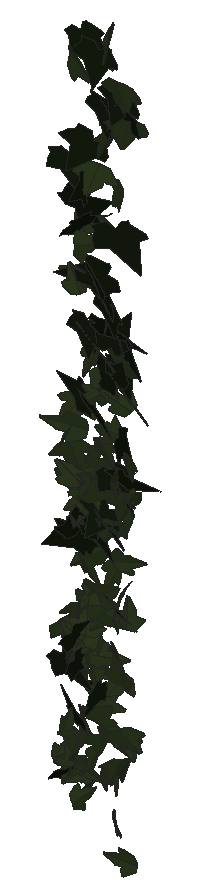
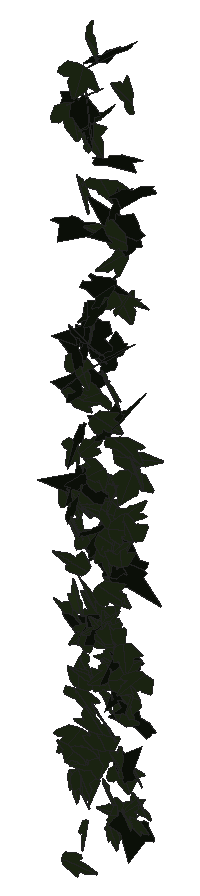
# SketchUp Ruby script. Lengths in inches.
U = 1.inch
M = Sketchup.active_model
def pt(a) = Geom::Point3d.new(a.map { |v| v * U })
def face(e, loops, mat)
  f = e.add_face(loops[0].map { |a| pt(a) })
  loops[1..].each { |l| e.add_face(l.map { |a| pt(a) }).erase! }
  f.material = f.back_material = mat if mat
  f
end
# faces: each face lists its corners as indices into pts; further lists are holes
def faces(e, pts, list, mat = nil) = list.each { |f| face(e, (f[0].is_a?(Array) ? f : [f]).map { |l| l.map { |i| pts[i] } }, mat) }
# xy, xz, yz: faces in a plane at the given z, y or x. An outline is a flat list of corners, or four numbers for a rectangle; further outlines are holes
def ring(l) = l.size == 4 ? [[l[0], l[1]], [l[2], l[1]], [l[2], l[3]], [l[0], l[3]]] : l.each_slice(2).to_a
def flat(e, list, mat, &to3) = list.each { |f| face(e, (f[0].is_a?(Array) ? f : [f]).map { |l| ring(l).map { |u, v| to3.(u, v) } }, mat) }
def xy(e, z, list, mat = nil) = flat(e, list, mat) { |x, y| [x, y, z] }
def xz(e, y, list, mat = nil) = flat(e, list, mat) { |x, z| [x, y, z] }
def yz(e, x, list, mat = nil) = flat(e, list, mat) { |y, z| [x, y, z] }
def lines(e, pts, list) = list.each { |a, b| e.add_line(pt(pts[a]), pt(pts[b])) }
# prism: a flat outline (further loops are holes) pulled along v
def prism(e, loops, v, mat = nil)
  f = face(e, loops, mat); d = Geom::Vector3d.new(v.map { |x| x * U })
  f.pushpull(f.normal.samedirection?(d) ? d.length : -d.length)
end
def box(e, o, s, mat = nil) = prism(e, [[o, [o[0] + s[0], o[1], o[2]], [o[0] + s[0], o[1] + s[1], o[2]], [o[0], o[1] + s[1], o[2]]]], [0, 0, s[2]], mat)
def at(x, y, z, deg = 0) = Geom::Transformation.translation(pt([x, y, z])) * Geom::Transformation.rotation(ORIGIN, Z_AXIS, deg.degrees)
def axes(o, x, y, z) = Geom::Transformation.new([*x, 0, *y, 0, *z, 0, *pt(o).to_a, 1])
def part(name) = M.definitions.add(name)
# library, detail: a bought-in or finely detailed component or shape, given as its bounding box
def library(name, o, s) = part(name).tap { |d| box(d.entities, o, s) }
def detail(e, o, s) = box(e.add_group.entities, o, s)
def put(e, d, t, mat = nil) = e.add_instance(d, t).tap { |i| i.material = mat if mat }
def group(e, t, mat = nil) = e.add_group.tap { |g| g.transformation = t; g.material = mat if mat }.entities
root = M.entities
M.materials.add("1026 AP 7946 SUNNY SIDE UP").color = [254, 231, 186]
M.materials.add("efeu1").color = [18, 25, 13]
M.materials.add("efeu2").color = [43, 57, 29]
c1 = part("ivyleaf_10")
p = [[0,0.5,-0.03],[-0.0625,2.02,-0.43],[-0.19,2.01,-0.46],[-0.54,1.05,-0.29],[-0.52,0.625,-0.18],[-0.83,0.76,-0.28],
  [-1.16,0.64,-0.33],[-1.15,0.33,-0.24],[-0.77,-0.39,0.02],[-0.3,-0.51,0.16],[0.04,-0.48,0.23],[-0.02,2.01,-0.4375],
  [-0.06,2.01,-0.43],[0.04,-0.49,0.23],[0.67,-0.49,0.14],[1.38,0.36,-0.2],[1.375,0.51,-0.24],[0.81,0.65,-0.19],
  [0.62,0.59,-0.15],[0.6,1.09,-0.28],[0.5,1.23,-0.31]]
faces(c1.entities,p,[[0,1,2,3,4,5,6,7,8,9,10],[11,12,0,13,14,15,16,17,18,19,20]],"efeu2")
c2 = part("ivyleaf_9")
p = [[1.54,2.16,1.25],[1.36,2.04,1.19],[-0.21,0.99,0.68],[-0.71,1.11,0.82],[-0.85,0.86,0.67],[-0.8,0.17,0.21],
  [-0.9,-0.01,0.1],[-0.67,-0.16,-0.02],[-0.08,-0.08,-0.05],[-0.03,-0.6,-0.4],[0.65,-0.88,-0.66],[0.83,-0.6,-0.49],
  [1.29,-0.42,-0.43],[1.8125,-0.07,-0.26],[1.21,0.44,0.15]]
faces(c2.entities,p,[[0,1,2,3,4,5,6,7,8,9,10,11,12,13,14]],"efeu1")
put(root,c1,axes([105.1,211.89,253.92],[0.25235,0.11815,0.14654],[-0.20286,-0.06215,0.20373],[0.20716,-0.20478,0.021]),"1026 AP 7946 SUNNY SIDE UP")
put(root,c2,axes([105.58,212.04,261.6],[0.04044,-0.21358,0.12299],[0.03918,-0.11835,-0.22211],[0.38367,0.0346,0.00972]),"1026 AP 7946 SUNNY SIDE UP")
put(root,c1,axes([105.06,211.72,250.5],[0.04226,0.045,-0.22259],[0.13994,0.19725,0.05482],[0.31799,-0.09279,0.00546]),"1026 AP 7946 SUNNY SIDE UP")
put(root,c2,axes([105.01,212.1,264.14],[0.00338,-0.11899,-0.23068],[0.24471,-0.17538,0.09682],[-0.31359,-0.13814,0.07306]),"1026 AP 7946 SUNNY SIDE UP")
put(root,c2,axes([105.33,212.05,267.23],[-0.1183,-0.24887,0.03019],[-0.00256,-0.03158,-0.26792],[0.39429,-0.07487,0.00732]),"1026 AP 7946 SUNNY SIDE UP")
put(root,c1,axes([104.97,211.93,251.83],[-0.2425,-0.13537,0.05546],[-0.04371,-0.05074,-0.21078],[0.22531,-0.15553,0.01879]),"1026 AP 7946 SUNNY SIDE UP")
put(root,c2,axes([105.14,212.04,259.25],[0.14991,-0.20524,0.14852],[0.09569,-0.13198,-0.23391],[0.38369,0.1131,0.00031]),"1026 AP 7946 SUNNY SIDE UP")
put(root,c2,axes([105.05,211.7,253.64],[0.00214,0.02141,-0.26801],[-0.22141,0.21927,0.01911],[0.34584,0.14024,0.01389]),"1026 AP 7946 SUNNY SIDE UP")
put(root,c2,axes([105.06,212.02,260.77],[0.20564,-0.18783,0.15192],[0.11526,-0.12971,-0.23623],[0.35845,0.14946,-0.01119]),"1026 AP 7946 SUNNY SIDE UP")
put(root,c2,axes([105.01,211.6875,263.38],[-0.03504,0.16493,-0.20943],[-0.03822,0.20278,0.17263],[0.41099,0.03292,-0.0018]),"1026 AP 7946 SUNNY SIDE UP")
put(root,c1,axes([104.89,211.97,258.68],[-0.0191,-0.02213,-0.2696],[-0.40694,-0.0428,0.01586],[-0.06906,0.25833,-0.0189]),"1026 AP 7946 SUNNY SIDE UP")
put(root,c1,axes([106,211.91,253.4],[-0.34779,0.05606,0.00791],[0.0193,0.0186,0.23418],[0.08678,0.22052,-0.02038]),"1026 AP 7946 SUNNY SIDE UP")
put(root,c1,axes([104.98,212,253.76],[0.20662,-0.06765,0.16385],[0.21278,-0.08479,-0.15246],[0.16995,0.1884,-0.00832]),"1026 AP 7946 SUNNY SIDE UP")
put(root,c1,axes([105.53,211.91,251.98],[-0.14705,-0.1867,-0.00857],[0.01832,0.00228,-0.21489],[0.29322,-0.09377,0.00913]),"1026 AP 7946 SUNNY SIDE UP")
put(root,c1,axes([105.96,211.76,257.87],[-0.04314,0.07268,0.21227],[-0.16295,0.17802,-0.07802],[-0.30176,-0.10653,0.01179]),"1026 AP 7946 SUNNY SIDE UP")
put(root,c1,axes([105.38,211.97,257.29],[-0.19438,-0.17108,-0.05241],[-0.06417,-0.03195,0.21678],[-0.27277,0.12943,-0.01365]),"1026 AP 7946 SUNNY SIDE UP")
put(root,c1,axes([104.66,211.9375,258.58],[0.12642,-0.22668,-0.02526],[-0.02371,0.01929,-0.24754],[0.35751,0.08143,-0.00749]),"1026 AP 7946 SUNNY SIDE UP")
put(root,c1,axes([106.25,211.89,249.42],[0.02755,-0.03254,-0.21439],[-0.31292,0.0653,-0.02742],[0.10763,0.19817,-0.02485]),"1026 AP 7946 SUNNY SIDE UP")
put(root,c2,axes([104.96,211.74,254.19],[-0.02593,0.01274,-0.26475],[-0.12622,0.24449,0.01922],[0.38452,0.08111,-0.01154]),"1026 AP 7946 SUNNY SIDE UP")
put(root,c2,axes([105.04,212.03,259.33],[0.03465,-0.26593,0.03037],[0.0179,0.032,0.27471],[-0.4206,-0.02054,0.01419]),"1026 AP 7946 SUNNY SIDE UP")
put(root,c1,axes([105.92,211.85,250.26],[-0.17709,0.1531,0.09478],[-0.10417,0.0641,-0.19491],[-0.26007,-0.12993,0.01353]),"1026 AP 7946 SUNNY SIDE UP")
put(root,c1,axes([105.19,212.1,254.97],[-0.0668,-0.06614,0.21725],[0.07074,-0.21321,-0.06069],[0.34082,0.03129,0.05518]),"1026 AP 7946 SUNNY SIDE UP")
put(root,c1,axes([105.68,211.81,251.22],[-0.05996,0.13436,0.16187],[-0.10001,0.14359,-0.14225],[-0.30835,-0.0727,0.01466]),"1026 AP 7946 SUNNY SIDE UP")
put(root,c1,axes([105.11,212,257.15],[0.24628,0.03322,-0.1483],[-0.21677,-0.04332,-0.16486],[-0.08432,0.2084,-0.00933]),"1026 AP 7946 SUNNY SIDE UP")
put(root,c2,axes([105.89,212.04,259.89],[0.23114,-0.19279,0.10579],[0.07883,-0.09205,-0.24984],[0.33513,0.15462,-0.0142]),"1026 AP 7946 SUNNY SIDE UP")
put(root,c1,axes([106.14,212.01,257.51],[-0.13584,-0.24496,0.05688],[-0.01308,-0.05703,-0.26769],[0.39511,-0.0861,0.0107]),"1026 AP 7946 SUNNY SIDE UP")
put(root,c1,axes([105.22,212.04,256.59],[-0.18532,0.08631,0.20308],[0.25445,-0.11176,0.1498],[0.22198,0.20016,-0.00217]),"1026 AP 7946 SUNNY SIDE UP")
put(root,c1,axes([104.76,211.92,258.22],[-0.27829,-0.18005,-0.08138],[0.10942,0.04059,-0.25902],[0.28847,-0.18909,0.01974]),"1026 AP 7946 SUNNY SIDE UP")
put(root,c2,axes([105.26,211.99,256.62],[0.18733,-0.20909,-0.04178],[-0.04724,0.02814,-0.24744],[0.3312,0.12228,-0.01166]),"1026 AP 7946 SUNNY SIDE UP")
put(root,c2,axes([105.48,212.15,256.95],[-0.20609,-0.19388,0.09948],[-0.05504,-0.09372,-0.2406],[0.33688,-0.13392,0.02154]),"1026 AP 7946 SUNNY SIDE UP")
put(root,c1,axes([106.0625,211.92,252.24],[-0.28277,-0.10075,-0.11678],[0.16761,0.03986,-0.21155],[0.16869,-0.2085,0.01444]),"1026 AP 7946 SUNNY SIDE UP")
put(root,c1,axes([106.11,211.96,258.42],[-0.25283,0.14617,-0.03396],[0.02008,-0.03602,-0.22332],[-0.23504,-0.16031,0.01745]),"1026 AP 7946 SUNNY SIDE UP")
put(root,c1,axes([105,212.04,255.71],[-0.16859,0.0918,-0.19613],[0.20692,-0.13881,-0.14571],[-0.26101,-0.16933,0.01117]),"1026 AP 7946 SUNNY SIDE UP")
put(root,c1,axes([104.99,212.1,250.97],[0.08817,0.06152,-0.2],[-0.16685,-0.16347,-0.08574],[-0.27393,0.11937,-0.01215]),"1026 AP 7946 SUNNY SIDE UP")
put(root,c1,axes([104.91,211.93,261.84],[0.0553,0.22951,-0.01182],[-0.02712,0.01552,0.23846],[0.36042,-0.03405,0.01976]),"1026 AP 7946 SUNNY SIDE UP")
put(root,c1,axes([104.44,211.96,251.12],[0.2897,-0.09034,-0.03767],[0.06401,0.00148,0.21049],[-0.1389,-0.18773,0.01844]),"1026 AP 7946 SUNNY SIDE UP")
put(root,c1,axes([104.59,211.96,251.8125],[0.26448,-0.12102,0.02234],[-0.0124,0.0272,0.21288],[-0.19312,-0.16749,0.01691]),"1026 AP 7946 SUNNY SIDE UP")
put(root,c2,axes([105.1,212.14,265.1],[-0.30262,-0.16331,0.03197],[-0.02123,-0.03337,-0.25967],[0.2608,-0.19222,0.01595]),"1026 AP 7946 SUNNY SIDE UP")
put(root,c1,axes([106.18,211.9375,254.76],[0.33082,-0.07285,0.08145],[-0.10332,0.05151,0.22815],[-0.13439,-0.21893,0.02508]),"1026 AP 7946 SUNNY SIDE UP")
put(root,c1,axes([104.96,212.03,262.08],[-0.32182,-0.05465,0.09783],[-0.12359,-0.06786,-0.21445],[0.12064,-0.21532,0.04129]),"1026 AP 7946 SUNNY SIDE UP")
put(root,c2,axes([105.91,211.87,260.04],[-0.01187,0.04313,0.27626],[-0.2037,0.23493,-0.04135],[-0.37493,-0.129,0.01372]),"1026 AP 7946 SUNNY SIDE UP")
put(root,c1,axes([105.85,212.05,251.45],[-0.12098,-0.20636,0.05195],[-0.01759,-0.05087,-0.22706],[0.334,-0.07743,0.00686]),"1026 AP 7946 SUNNY SIDE UP")
put(root,c2,axes([105.82,212.03,263.39],[-0.12215,-0.19003,-0.20318],[0.20299,0.15416,-0.20563],[0.37843,-0.14403,0.04472]),"1026 AP 7946 SUNNY SIDE UP")
put(root,c1,axes([106.03,211.89,257.47],[0.07328,-0.09,-0.20202],[-0.14802,0.17145,-0.10338],[0.30446,0.10502,-0.00164]),"1026 AP 7946 SUNNY SIDE UP")
put(root,c1,axes([104.78,212.04,257.45],[0.11128,0.18827,0.10955],[-0.10232,-0.08699,0.20484],[0.32337,-0.09232,0.02712]),"1026 AP 7946 SUNNY SIDE UP")
put(root,c2,axes([104.83,212.05,256.26],[0.28183,0.10185,0.15873],[-0.23932,-0.03878,0.20937],[0.16319,-0.23277,0.03291]),"1026 AP 7946 SUNNY SIDE UP")
put(root,c2,axes([104.87,212.04,256.25],[0.0613,0.01181,-0.2616],[-0.31834,-0.15404,-0.04029],[-0.24192,0.20569,-0.01327]),"1026 AP 7946 SUNNY SIDE UP")
put(root,c1,axes([105.38,212,252.3],[-0.28879,-0.05589,0.08349],[0.11178,0.04436,0.19696],[-0.10769,0.19592,-0.01947]),"1026 AP 7946 SUNNY SIDE UP")
put(root,c1,axes([105.5,212.02,257.98],[0.17335,0.01351,-0.18872],[-0.28876,0.01569,-0.11253],[0.01027,0.21329,0.02149]),"1026 AP 7946 SUNNY SIDE UP")
put(root,c1,axes([105.73,212.14,251.16],[0.13532,-0.08406,0.19964],[0.20446,-0.14448,-0.1246],[0.26263,0.15579,-0.00586]),"1026 AP 7946 SUNNY SIDE UP")
put(root,c2,axes([105.48,212.08,262.25],[-0.07815,-0.06548,-0.2621],[-0.31174,-0.15997,0.08149],[-0.27017,0.20352,-0.01822]),"1026 AP 7946 SUNNY SIDE UP")
put(root,c1,axes([105.36,212.01,254.07],[0.19498,-0.14721,-0.06661],[-0.08174,0.03945,-0.19756],[0.23869,0.13376,-0.01324]),"1026 AP 7946 SUNNY SIDE UP")
put(root,c1,axes([105.58,212.1,265.44],[0.00003,-0.24196,0.08798],[0.00904,-0.08675,-0.24971],[0.40409,0.00196,0.00558]),"1026 AP 7946 SUNNY SIDE UP")
put(root,c1,axes([105.79,212.13,256.78],[0.01121,0.00261,0.22185],[0.27602,-0.12487,-0.00515],[0.19614,0.17557,-0.00542]),"1026 AP 7946 SUNNY SIDE UP")
put(root,c1,axes([105.67,212.07,256.71],[-0.20084,-0.17707,0.06693],[-0.04057,-0.06254,-0.22476],[0.29434,-0.12944,0.01469]),"1026 AP 7946 SUNNY SIDE UP")
put(root,c1,axes([106.05,212.02,259.52],[0.12715,0.08011,0.19605],[-0.30285,-0.04311,0.103],[0.11518,-0.2018,0.05441]),"1026 AP 7946 SUNNY SIDE UP")
put(root,c1,axes([105.92,212.01,266.62],[-0.41779,0.056,-0.01286],[0.01121,-0.02793,-0.27863],[-0.08963,-0.26454,0.02507]),"1026 AP 7946 SUNNY SIDE UP")
put(root,c1,axes([105.375,212.02,255.03],[-0.30387,-0.0059,0.15661],[0.23593,0.03358,0.19799],[-0.03989,0.2436,-0.02204]),"1026 AP 7946 SUNNY SIDE UP")
put(root,c1,axes([105.1,211.96,254.22],[0.26814,0.11094,-0.0378],[0.03181,0.03702,0.20882],[0.18127,-0.1706,0.01926]),"1026 AP 7946 SUNNY SIDE UP")
put(root,c2,axes([105.98,211.92,258.82],[0.11893,-0.10032,-0.22469],[-0.24995,0.14965,-0.12715],[0.2818,0.17507,-0.01796]),"1026 AP 7946 SUNNY SIDE UP")
put(root,c1,axes([105.22,212.06,251.41],[0.20534,-0.18634,-0.01108],[-0.02534,0.00053,-0.23403],[0.2923,0.13095,-0.0125]),"1026 AP 7946 SUNNY SIDE UP")
put(root,c2,axes([105.18,212.2,262.11],[0.05129,-0.18678,0.16592],[0.03044,-0.16109,-0.19616],[0.3877,0.03736,-0.00655]),"1026 AP 7946 SUNNY SIDE UP")
put(root,c1,axes([105.13,212.18,257.48],[-0.00855,-0.14831,0.18277],[0.01088,-0.17833,-0.15367],[0.36445,0.00185,0.00887]),"1026 AP 7946 SUNNY SIDE UP")
put(root,c2,axes([104.8,212.0625,263.54],[-0.04297,0.00442,0.27365],[0.33607,-0.1582,0.02444],[0.24806,0.2151,0.01429]),"1026 AP 7946 SUNNY SIDE UP")
put(root,c1,axes([104.82,212.16,252.08],[-0.00652,-0.02193,0.25281],[0.31686,-0.14172,-0.01036],[0.22323,0.20053,0.02209]),"1026 AP 7946 SUNNY SIDE UP")
put(root,c1,axes([105.37,211.95,253.27],[0.20921,-0.05886,0.16909],[-0.22129,0.08636,0.14963],[-0.16271,-0.19312,0.01391]),"1026 AP 7946 SUNNY SIDE UP")
put(root,c1,axes([105.03,211.85,262.88],[0.0403,-0.07202,-0.27758],[0.17967,0.24911,-0.05603],[0.39938,-0.1048,0.05321]),"1026 AP 7946 SUNNY SIDE UP")
put(root,c1,axes([105.86,211.92,254.7],[-0.07748,0.06406,0.20105],[-0.22873,0.13029,-0.08129],[-0.22727,-0.15297,0.01326]),"1026 AP 7946 SUNNY SIDE UP")
put(root,c1,axes([105.85,212.16,255.18],[0.02025,-0.17893,-0.15143],[0.0685,-0.1417,0.18206],[-0.35659,-0.03738,0.02637]),"1026 AP 7946 SUNNY SIDE UP")
put(root,c1,axes([105.34,211.9,254.875],[0.02003,-0.08057,-0.22542],[0.18826,0.1898,-0.06384],[0.31384,-0.10871,0.05268]),"1026 AP 7946 SUNNY SIDE UP")
put(root,c1,axes([105.55,212.2,254.64],[-0.09839,-0.11212,0.20362],[-0.04408,-0.20028,-0.12695],[0.35546,-0.05587,0.04062]),"1026 AP 7946 SUNNY SIDE UP")
put(root,c2,axes([105.32,212.14,252.97],[-0.29183,0.05244,-0.15979],[0.22168,-0.06891,-0.19782],[-0.13178,-0.23205,0.02109]),"1026 AP 7946 SUNNY SIDE UP")
put(root,c1,axes([105.32,212.03,253.7],[0.05672,-0.05653,-0.23259],[0.36473,-0.0058,0.0397],[-0.02332,-0.22825,0.05518]),"1026 AP 7946 SUNNY SIDE UP")
put(root,c1,axes([104.5625,212.2,251.23],[-0.06575,0.03333,0.21213],[0.05752,-0.20539,0.04074],[0.32261,0.04341,0.03597]),"1026 AP 7946 SUNNY SIDE UP")
put(root,c1,axes([105.88,211.92,253.84],[0.00269,-0.03311,-0.23354],[-0.17366,0.19829,-0.02956],[0.31528,0.1095,-0.01429]),"1026 AP 7946 SUNNY SIDE UP")
put(root,c1,axes([105.08,212.15,258.09],[-0.14379,0.08128,-0.17796],[0.1412,-0.15128,-0.12286],[-0.26565,-0.1244,0.03102]),"1026 AP 7946 SUNNY SIDE UP")
put(root,c2,axes([104.95,212.2,260.94],[-0.03941,-0.23865,0.04555],[0.00361,-0.04604,-0.24738],[0.38202,-0.02418,0.00704]),"1026 AP 7946 SUNNY SIDE UP")
put(root,c2,axes([105.84,212.1875,260.77],[0.03744,-0.03995,-0.27471],[0.41466,-0.05126,0.0319],[-0.08666,-0.26253,0.03394]),"1026 AP 7946 SUNNY SIDE UP")
put(root,c2,axes([105.35,212.05,261.09],[0.34249,-0.05913,0.14579],[0.20596,-0.05727,-0.23212],[0.12639,0.25354,-0.01679]),"1026 AP 7946 SUNNY SIDE UP")
put(root,c1,axes([105.24,212.11,264.5],[0.36808,0.08143,-0.05917],[-0.0728,-0.04231,-0.25437],[-0.13923,0.2374,-0.02344]),"1026 AP 7946 SUNNY SIDE UP")
put(root,c2,axes([104.54,212.13,264.59],[-0.07047,-0.22834,-0.09463],[0.04717,0.08628,-0.2389],[0.38336,-0.05259,0.012]),"1026 AP 7946 SUNNY SIDE UP")
put(root,c1,axes([106.05,212.09,265.78],[-0.35177,-0.15134,0.04593],[-0.03926,-0.04392,-0.27757],[0.24534,-0.22402,0.02144]),"1026 AP 7946 SUNNY SIDE UP")
put(root,c1,axes([105.87,212.04,255.97],[-0.12565,-0.01491,0.19577],[0.2761,0.07467,0.0825],[-0.11698,0.19224,-0.01556]),"1026 AP 7946 SUNNY SIDE UP")
put(root,c2,axes([105.71,212.04,257.93],[0.02855,-0.18953,-0.17885],[-0.04376,0.17048,-0.19495],[0.40061,0.03213,-0.00855]),"1026 AP 7946 SUNNY SIDE UP")
put(root,c1,axes([105.08,212.1,254.79],[-0.02205,-0.23591,0.00415],[0.00944,0.00502,0.24342],[-0.37091,0.01415,0.00595]),"1026 AP 7946 SUNNY SIDE UP")
put(root,c1,axes([104.85,212.07,253.11],[-0.30088,0.08192,-0.03889],[-0.04726,0.02673,0.2142],[0.13405,0.19329,-0.01178]),"1026 AP 7946 SUNNY SIDE UP")
put(root,c1,axes([104.81,211.99,256.74],[-0.01847,0.20215,0.08432],[-0.02911,0.0796,-0.20771],[-0.34101,-0.01775,0.01316]),"1026 AP 7946 SUNNY SIDE UP")
put(root,c1,axes([104.77,212.09,251],[0.05721,0.0064,0.22846],[0.34702,0.02156,-0.03783],[-0.03509,0.22366,-0.00157]),"1026 AP 7946 SUNNY SIDE UP")
put(root,c1,axes([105.15,212.23,256.91],[-0.07658,-0.15946,0.1852],[-0.03013,-0.18118,-0.17111],[0.37772,-0.04678,0.0239]),"1026 AP 7946 SUNNY SIDE UP")
put(root,c1,axes([104.57,212.14,251.01],[0.33387,-0.08953,0.01993],[0.01601,-0.02675,-0.2366],[0.1433,0.21157,-0.02]),"1026 AP 7946 SUNNY SIDE UP")
put(root,c2,axes([105.28,212.17,256.8],[0.21387,-0.19136,0.06303],[0.04101,-0.05776,-0.24189],[0.31376,0.13799,-0.01135]),"1026 AP 7946 SUNNY SIDE UP")
put(root,c2,axes([105.32,212.27,265.9],[-0.01648,-0.23207,0.11736],[0.02769,-0.11571,-0.23907],[0.40647,-0.00153,0.02104]),"1026 AP 7946 SUNNY SIDE UP")
put(root,c1,axes([104.64,212.2,251.16],[0.12002,-0.17241,0.12161],[0.07828,-0.10812,-0.19488],[0.32,0.09112,0.00206]),"1026 AP 7946 SUNNY SIDE UP")
put(root,c1,axes([105.86,212.05,264.26],[0.21086,-0.18897,-0.11164],[-0.06424,0.10191,-0.2369],[0.33559,0.13824,0.02479]),"1026 AP 7946 SUNNY SIDE UP")
put(root,c1,axes([104.93,212.09,263.41],[0.02498,0.02074,0.26953],[0.40848,0.03522,-0.01893],[-0.05741,0.25962,-0.01741]),"1026 AP 7946 SUNNY SIDE UP")
put(root,c1,axes([105.05,212.1,257.83],[-0.11633,0.19647,-0.0431],[0.01214,-0.04295,-0.21638],[-0.316,-0.07398,0.00755]),"1026 AP 7946 SUNNY SIDE UP")
put(root,c1,axes([105.84,212.14,253.3],[0.34425,-0.03338,-0.06796],[-0.10717,-0.01279,-0.2271],[0.04435,0.22824,-0.0213]),"1026 AP 7946 SUNNY SIDE UP")
put(root,c1,axes([105.11,211.98,253.97],[-0.10871,-0.10036,-0.20933],[0.21394,0.15077,-0.12388],[0.28398,-0.152,0.01319]),"1026 AP 7946 SUNNY SIDE UP")
put(root,c2,axes([105.51,212.18,265.53],[-0.04102,0.14763,0.23261],[-0.04825,-0.22617,0.14791],[0.42032,-0.01155,0.03968]),"1026 AP 7946 SUNNY SIDE UP")
put(root,c1,axes([105.07,212.13,250.65],[0.01849,-0.20578,0.01115],[0.00018,-0.01201,-0.21241],[0.32412,0.01175,-0.00052]),"1026 AP 7946 SUNNY SIDE UP")
put(root,c2,axes([105.58,211.98,257.78],[0.13459,0.09069,-0.24366],[0.21732,0.19315,0.12868],[0.33469,-0.16188,0.01443]),"1026 AP 7946 SUNNY SIDE UP")
put(root,c1,axes([105.62,212.04,254.67],[-0.17573,-0.0929,-0.14883],[0.19606,0.07375,-0.14834],[0.18473,-0.16664,0.01586]),"1026 AP 7946 SUNNY SIDE UP")
put(root,c2,axes([104.91,212.09,267.51],[0.12738,-0.21814,-0.13302],[0.01509,0.13684,-0.23341],[0.39732,0.06474,0.05151]),"1026 AP 7946 SUNNY SIDE UP")
put(root,c2,axes([105.55,212.27,261.03],[0.11386,-0.06656,-0.25837],[0.36744,-0.09558,0.09522],[-0.17605,-0.24253,0.03163]),"1026 AP 7946 SUNNY SIDE UP")
put(root,c2,axes([105.43,212.22,254.77],[0.16226,-0.13408,0.19737],[0.17003,-0.15925,-0.17506],[0.32713,0.14928,-0.00691]),"1026 AP 7946 SUNNY SIDE UP")
put(root,c1,axes([104.46,212.2,253.71],[-0.11145,0.0527,-0.21378],[0.23135,-0.14724,-0.09103],[-0.2452,-0.16288,0.01128]),"1026 AP 7946 SUNNY SIDE UP")
put(root,c1,axes([106.04,212.12,256.92],[0.17656,-0.18833,-0.04229],[-0.04891,0.02793,-0.22536],[0.29875,0.11587,-0.0119]),"1026 AP 7946 SUNNY SIDE UP")
put(root,c1,axes([105.66,212.17,255.6875],[0.28995,-0.17068,0.01088],[-0.00672,-0.02154,-0.25826],[0.2689,0.1835,-0.01818]),"1026 AP 7946 SUNNY SIDE UP")
put(root,c1,axes([105.59,212.23,258.67],[0.01524,0.13924,0.18412],[-0.00148,-0.17807,0.14257],[0.35526,-0.00672,-0.00731]),"1026 AP 7946 SUNNY SIDE UP")
put(root,c1,axes([104.76,212.12,254.58],[-0.11749,-0.20882,-0.0195],[0.01827,0.01468,-0.22831],[0.32902,-0.07538,0.00572]),"1026 AP 7946 SUNNY SIDE UP")
put(root,c2,axes([105.27,212.3,261.74],[0.07585,-0.19485,0.17183],[0.04052,-0.16631,-0.20743],[0.40241,0.05347,-0.0115]),"1026 AP 7946 SUNNY SIDE UP")
put(root,c2,axes([104.37,212.17,253.29],[-0.03387,-0.07884,-0.2405],[0.36058,0.07819,-0.04864],[0.13994,-0.22055,0.06711]),"1026 AP 7946 SUNNY SIDE UP")
put(root,c1,axes([105.45,212.28,267.59],[0.18019,-0.18298,0.20829],[0.17275,-0.17097,-0.22341],[0.39376,0.15874,0.0027]),"1026 AP 7946 SUNNY SIDE UP")
put(root,c1,axes([105.34,212.17,259.95],[0.28071,-0.00185,0.18092],[0.2742,-0.02797,-0.18308],[0.03291,0.24886,-0.01776]),"1026 AP 7946 SUNNY SIDE UP")
put(root,c1,axes([105.41,212.08,252.64],[0.37266,-0.03667,-0.06615],[0.1054,0.01717,0.24567],[-0.04841,-0.24489,0.02566]),"1026 AP 7946 SUNNY SIDE UP")
put(root,c1,axes([105.25,212.24,259.45],[-0.13593,-0.10015,0.17482],[-0.10735,-0.15925,-0.13314],[0.29146,-0.10536,0.03249]),"1026 AP 7946 SUNNY SIDE UP")
put(root,c2,axes([104.78,212.12,251.98],[0.1222,-0.15866,0.17253],[-0.07958,0.16165,0.18194],[-0.35496,-0.09087,0.0186]),"1026 AP 7946 SUNNY SIDE UP")
put(root,c2,axes([105.74,212.33,266.22],[-0.14664,-0.20724,0.12479],[-0.00173,-0.1308,-0.22996],[0.37838,-0.08091,0.04731]),"1026 AP 7946 SUNNY SIDE UP")
put(root,c1,axes([104.56,212.15,257.19],[-0.31318,0.00427,0.12969],[0.19802,0.00545,0.20514],[0.00109,0.23554,-0.00572]),"1026 AP 7946 SUNNY SIDE UP")
put(root,c1,axes([104.43,212.06,254.06],[-0.16845,-0.13097,-0.16382],[0.20751,0.09293,-0.17069],[0.24756,-0.16701,0.03161]),"1026 AP 7946 SUNNY SIDE UP")
put(root,c1,axes([105.99,212.13,251.43],[0.02652,-0.22694,-0.03861],[-0.00513,0.03605,-0.23423],[0.36132,0.01717,-0.00049]),"1026 AP 7946 SUNNY SIDE UP")
put(root,c1,axes([104.5,212.28,253.47],[-0.01351,0.02829,0.22158],[0.16594,-0.18733,0.02865],[0.29774,0.10569,-0.00592]),"1026 AP 7946 SUNNY SIDE UP")
put(root,c1,axes([105.59,211.99,261.48],[0.12268,-0.15013,-0.22722],[-0.02429,0.22601,-0.16343],[0.41771,0.05723,0.05723]),"1026 AP 7946 SUNNY SIDE UP")
put(root,c2,axes([105.68,212.04,260.74],[-0.27222,0.16083,0.08997],[0.12137,-0.04346,0.24235],[0.26016,0.18855,-0.01892]),"1026 AP 7946 SUNNY SIDE UP")
put(root,c1,axes([105.91,212.1,260.44],[-0.30344,0.05602,0.14254],[-0.21839,0.01406,-0.20582],[-0.08474,-0.23685,0.02002]),"1026 AP 7946 SUNNY SIDE UP")
put(root,c1,axes([105.49,212.3,265.4],[-0.07853,0.10794,0.24797],[0.20254,-0.20309,0.12048],[0.36097,0.13743,-0.01366]),"1026 AP 7946 SUNNY SIDE UP")
put(root,c2,axes([104.57,212.02,250.86],[0.13256,0.22787,0.00315],[0.01242,-0.00104,-0.25018],[-0.3581,0.08432,-0.00751]),"1026 AP 7946 SUNNY SIDE UP")
put(root,c1,axes([105.52,212.17,252],[-0.26126,0.04098,-0.16915],[0.23539,-0.07241,-0.17485],[-0.12485,-0.22226,0.02429]),"1026 AP 7946 SUNNY SIDE UP")
put(root,c1,axes([105.92,212.2,251.99],[0.27669,-0.00875,0.12237],[0.18259,-0.03491,-0.18],[0.04199,0.20944,-0.02363]),"1026 AP 7946 SUNNY SIDE UP")
put(root,c1,axes([105.11,212.26,255.82],[-0.15672,-0.10029,0.18359],[-0.15526,-0.15072,-0.1447],[0.28246,-0.13849,0.02233]),"1026 AP 7946 SUNNY SIDE UP")
put(root,c1,axes([104.79,212.2,256.56],[-0.11989,-0.19427,-0.03481],[-0.02963,-0.0277,0.2147],[-0.30834,0.0782,-0.00709]),"1026 AP 7946 SUNNY SIDE UP")
put(root,c1,axes([104.78,212.21,259.125],[0.34496,0.00704,-0.11633],[-0.1745,-0.035,-0.22449],[-0.03494,0.24426,-0.02735]),"1026 AP 7946 SUNNY SIDE UP")
put(root,c1,axes([104.83,212.32,254.01],[-0.00712,-0.04197,0.21189],[0.02092,-0.20561,-0.04407],[0.32978,0.01214,0.00737]),"1026 AP 7946 SUNNY SIDE UP")
put(root,c2,axes([105.87,212.1,266.03],[0.23348,0.01706,-0.2393],[-0.35666,-0.05247,-0.15359],[-0.08383,0.27073,-0.01304]),"1026 AP 7946 SUNNY SIDE UP")
put(root,c2,axes([105.71,212.27,260.24],[0.0529,-0.24673,0.01069],[0.00037,-0.01185,-0.25659],[0.3884,0.03362,-0.00121]),"1026 AP 7946 SUNNY SIDE UP")
put(root,c1,axes([105.06,212.13,254.72],[-0.25952,-0.06343,0.14163],[0.18649,0.0731,0.18139],[-0.14881,0.20223,-0.01969]),"1026 AP 7946 SUNNY SIDE UP")
put(root,c1,axes([105.05,212.23,260.31],[0.2738,-0.18211,0.04498],[0.02644,-0.04558,-0.25909],[0.29366,0.1739,-0.01861]),"1026 AP 7946 SUNNY SIDE UP")
put(root,c2,axes([105.85,212.35,257.27],[-0.0033,-0.06673,0.24295],[-0.00584,-0.23618,-0.07015],[0.38591,-0.00414,0.00101]),"1026 AP 7946 SUNNY SIDE UP")
put(root,c1,axes([104.5,212.29,266.65],[0.0207,-0.02094,0.29756],[0.40686,-0.12928,-0.02255],[0.20494,0.25877,0.01472]),"1026 AP 7946 SUNNY SIDE UP")
put(root,c1,axes([105.29,212.21,258.34],[-0.2413,0.08643,-0.14283],[0.15772,-0.10114,-0.17929],[-0.20361,-0.18077,0.03039]),"1026 AP 7946 SUNNY SIDE UP")
put(root,c1,axes([105.13,212.19,256.64],[-0.12583,-0.2106,0.00404],[0.00956,-0.00778,-0.23198],[0.33111,-0.07981,0.00823]),"1026 AP 7946 SUNNY SIDE UP")
put(root,c1,axes([104.8125,212.33,257.27],[0.01465,-0.06364,0.20744],[0.0162,-0.20154,-0.06717],[0.3322,0.01264,-0.00587]),"1026 AP 7946 SUNNY SIDE UP")
put(root,c1,axes([105.89,212.19,257.59],[0.29377,-0.07052,-0.09112],[-0.13562,0.02051,-0.20533],[0.11433,0.20552,-0.00942]),"1026 AP 7946 SUNNY SIDE UP")
put(root,c1,axes([105.02,212.14,257.43],[-0.01247,-0.00748,0.21922],[0.30848,0.08262,0.01101],[-0.13031,0.19631,0.00507]),"1026 AP 7946 SUNNY SIDE UP")
